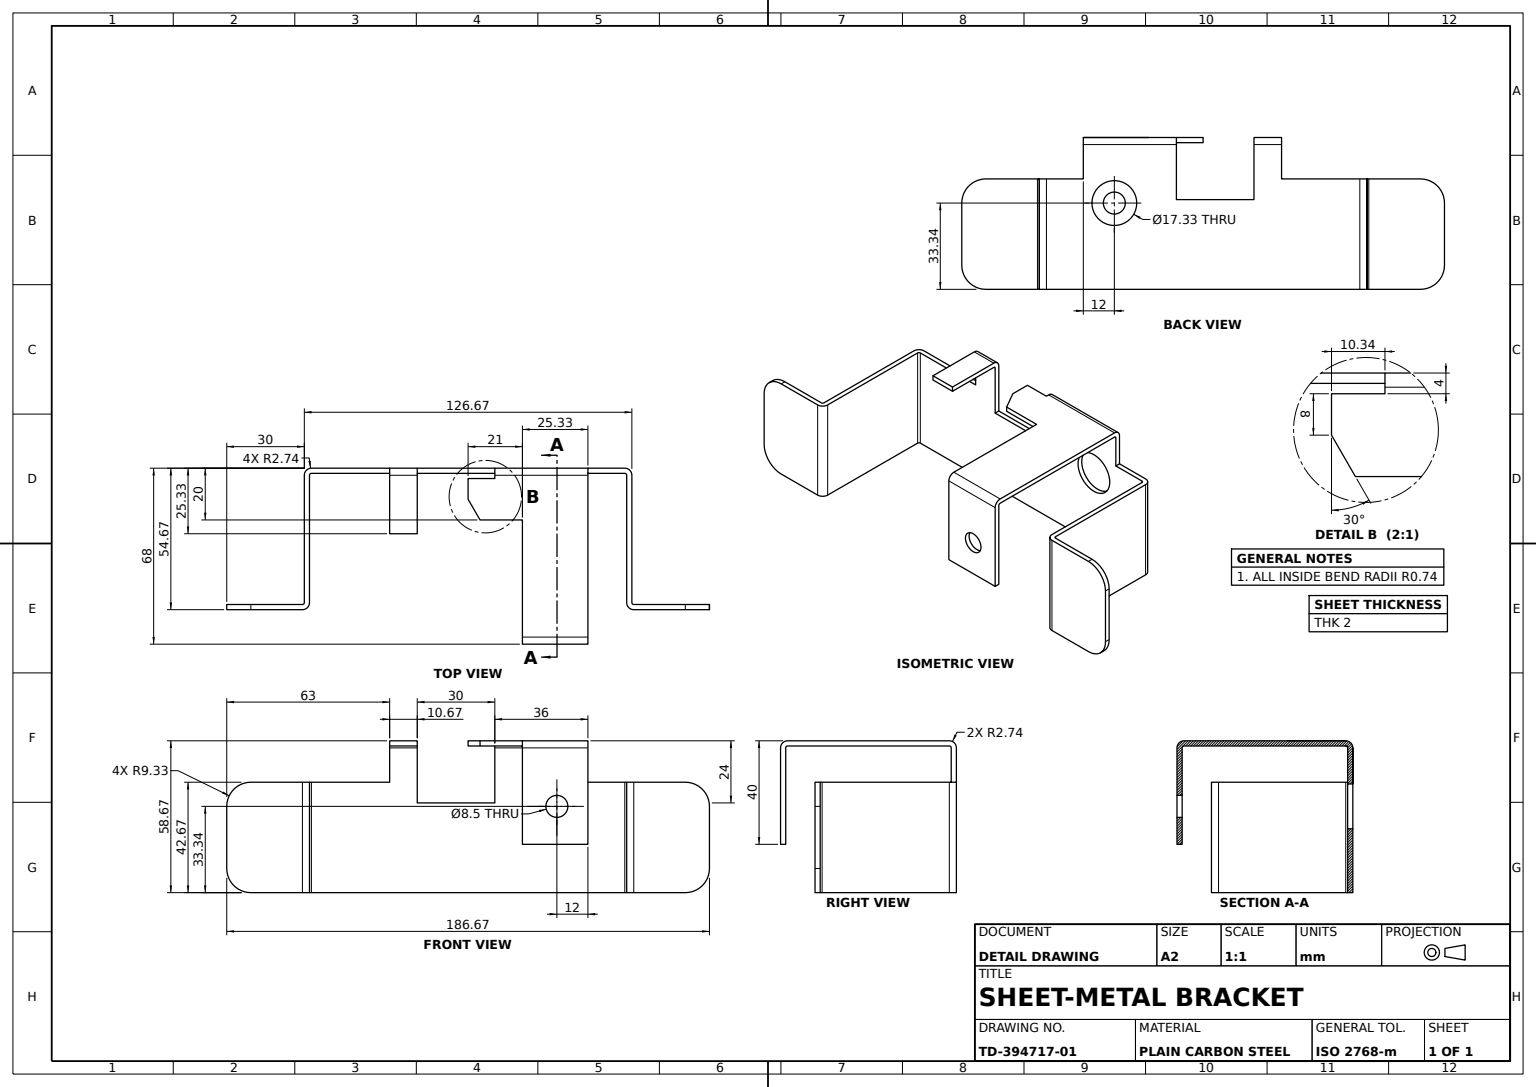
solid
v1 (10.335,13.335,-2)
v2 (10.335,13.335,0)
e1 v1 v2 LINE
v3 (-19.665,13.335,-2)
e2 v1 v3 LINE
v4 (-19.665,13.335,0)
e3 v3 v4 LINE
e4 v4 v2 LINE
face PLANE(AX(P(10.335,13.335,-58),D(0,-1,0),D(1,0,0))) rev [-e1 e2 e3 e4]
v5 (63.335,21.335,49.9334)
v6 (64.0716,21.335,50.67)
e5 v5 v6 CIRCLE(AX(P(64.0716,21.335,49.9334),D(0,1,0),D(0,0,-1)),0.7366)
v7 (64.0716,-21.335,50.67)
e6 v6 v7 LINE
v8 (63.335,-21.335,49.9334)
e7 v7 v8 CIRCLE(AX(P(64.0716,-21.335,49.9334),D(0,-1,0),D(0,0,-1)),0.7366)
e8 v8 v5 LINE
face CYL(AX(P(64.0716,-21.335,49.9334),D(0,-1,0),D(0,0,1)),0.7366) rev [e5 e6 e7 e8]
v9 (-84.005,-21.335,52.67)
v10 (-84.005,-21.335,50.67)
e9 v9 v10 LINE
v11 (-93.335,-12.005,52.67)
e10 v11 v9 CIRCLE(AX(P(-84.005,-12.005,52.67),D(0,0,1),D(1,0,0)),9.33)
v12 (-93.335,-12.005,50.67)
e11 v12 v11 LINE
e12 v10 v12 CIRCLE(AX(P(-84.005,-12.005,50.67),D(0,0,-1),D(1,0,0)),9.33)
face CYL(AX(P(-84.005,-12.005,52.67),D(0,0,-1),D(-1,0,0)),9.33) [-e9 -e10 -e11 -e12]
v13 (46.335,34.5984,66)
v14 (21.005,34.5984,66)
e13 v13 v14 LINE
v15 (46.335,37.335,63.2634)
e14 v15 v13 CIRCLE(AX(P(46.335,34.5984,63.2634),D(1,0,0),D(0,0,1)),2.7366)
v16 (21.005,37.335,63.2634)
e15 v16 v15 LINE
e16 v14 v16 CIRCLE(AX(P(21.005,34.5984,63.2634),D(-1,0,0),D(0,0,-1)),2.7366)
face CYL(AX(P(10.335,34.5984,63.2634),D(-1,0,0),D(0,0,1)),2.7366) [-e13 -e14 -e15 -e16]
v17 (38.585,12.005,64)
v18 (38.585,12.005,66)
e17 v17 v18 LINE
v19 (30.085,12.005,66)
e18 v18 v19 CIRCLE(AX(P(34.335,12.005,66),D(0,0,1),D(1,0,0)),4.25)
v20 (30.085,12.005,64)
e19 v20 v19 LINE
e20 v17 v20 CIRCLE(AX(P(34.335,12.005,64),D(0,0,1),D(0,-1,0)),4.25)
face CYL(AX(P(34.335,12.005,62),D(0,0,1),D(1,0,0)),4.25) rev [e17 e18 -e19 -e20]
v21 (61.335,21.335,0.7366)
v22 (60.5984,21.335,0)
e21 v21 v22 CIRCLE(AX(P(60.5984,21.335,0.7366),D(0,1,0),D(0,0,1)),0.7366)
v23 (63.335,21.335,0.7366)
e22 v21 v23 LINE
v24 (60.5984,21.335,-2)
e23 v23 v24 CIRCLE(AX(P(60.5984,21.335,0.7366),D(0,1,0),D(0,0,1)),2.7366)
e24 v22 v24 LINE
face PLANE(AX(P(60.5984,21.335,0.7366),D(0,-1,0),D(0,0,-1))) rev [-e21 e22 e23 -e24]
v25 (-64.0716,-21.335,50.67)
e25 v25 v10 LINE
v26 (-93.335,12.005,50.67)
e26 v12 v26 LINE
v27 (-84.005,21.335,50.67)
e27 v26 v27 CIRCLE(AX(P(-84.005,12.005,50.67),D(0,0,-1),D(1,0,0)),9.33)
v28 (-64.0716,21.335,50.67)
e28 v27 v28 LINE
e29 v25 v28 LINE
face PLANE(AX(P(0,0,50.67),D(0,0,1),D(1,0,0))) rev [e25 e12 e26 e27 e28 -e29]
v29 (-30.335,37.335,0.7366)
v30 (-30.335,37.335,23.33)
e30 v29 v30 LINE
v31 (-19.665,37.335,23.33)
e31 v30 v31 LINE
v32 (-19.665,37.335,0.7366)
e32 v31 v32 LINE
e33 v29 v32 LINE
face PLANE(AX(P(0,37.335,0),D(0,-1,0),D(0,0,-1))) rev [e30 e31 e32 -e33]
v33 (-84.005,21.335,52.67)
e34 v27 v33 LINE
v34 (-93.335,12.005,52.67)
e35 v34 v26 LINE
e36 v33 v34 CIRCLE(AX(P(-84.005,12.005,52.67),D(0,0,1),D(1,0,0)),9.33)
face CYL(AX(P(-84.005,12.005,52.67),D(0,0,-1),D(-1,0,0)),9.33) [-e34 -e27 -e35 -e36]
v35 (61.335,21.335,49.9334)
e37 v21 v35 LINE
e38 v5 v35 LINE
e39 v23 v5 LINE
face PLANE(AX(P(63.335,21.335,52.67),D(0,-1,0),D(0,0,-1))) rev [e37 -e38 -e39 -e22]
v36 (25.67,12.005,-2)
v37 (43,12.005,-2)
e40 v36 v37 CIRCLE(AX(P(34.335,12.005,-2),D(0,0,-1),D(-1,0,0)),8.665)
e41 v37 v36 CIRCLE(AX(P(34.335,12.005,-2),D(0,0,-1),D(-1,0,0)),8.665)
v38 (10.335,34.5984,-2)
v39 (46.335,34.5984,-2)
e42 v38 v39 LINE
v40 (46.335,21.335,-2)
e43 v40 v39 LINE
e44 v24 v40 LINE
v41 (60.5984,-21.335,-2)
e45 v24 v41 LINE
v42 (-60.5984,-21.335,-2)
e46 v42 v41 LINE
v43 (-60.5984,21.335,-2)
e47 v42 v43 LINE
v44 (-30.335,21.335,-2)
e48 v44 v43 LINE
v45 (-30.335,34.5984,-2)
e49 v45 v44 LINE
v46 (-19.665,34.5984,-2)
e50 v45 v46 LINE
e51 v3 v46 LINE
e52 v38 v1 LINE
face PLANE(AX(P(0,0,-2),D(0,0,-1),D(-1,0,0))) [-e40 -e41] [e42 -e43 -e44 e45 -e46 e47 -e48 -e49 e50 -e51 -e2 -e52]
v47 (10.335,37.335,0.7366)
v48 (46.335,37.335,0.7366)
e53 v47 v48 LINE
v49 (10.335,37.335,2)
e54 v49 v47 LINE
v50 (0,37.335,2)
e55 v50 v49 LINE
v51 (0,37.335,10)
e56 v51 v50 LINE
v52 (4.618802,37.335,18)
e57 v51 v52 LINE
v53 (21.005,37.335,18)
e58 v53 v52 LINE
e59 v53 v16 LINE
e60 v15 v48 LINE
face PLANE(AX(P(0,37.335,0),D(0,-1,0),D(0,0,-1))) rev [-e53 -e54 -e55 -e56 e57 -e58 e59 e15 e60]
v54 (93.335,12.005,52.67)
v55 (84.005,21.335,52.67)
e61 v54 v55 CIRCLE(AX(P(84.005,12.005,52.67),D(0,0,1),D(-1,0,0)),9.33)
v56 (64.0716,21.335,52.67)
e62 v55 v56 LINE
v57 (64.0716,-21.335,52.67)
e63 v57 v56 LINE
v58 (84.005,-21.335,52.67)
e64 v57 v58 LINE
v59 (93.335,-12.005,52.67)
e65 v58 v59 CIRCLE(AX(P(84.005,-12.005,52.67),D(0,0,1),D(-1,0,0)),9.33)
e66 v59 v54 LINE
face PLANE(AX(P(0,0,52.67),D(0,0,-1),D(-1,0,0))) rev [e61 e62 -e63 e64 e65 e66]
v60 (0,35.335,2)
e67 v50 v60 LINE
v61 (0,35.335,10)
e68 v61 v60 LINE
e69 v61 v51 LINE
face PLANE(AX(P(0,37.335,8),D(-1,0,0),D(0,0,1))) [e67 -e68 e69 e56]
v62 (46.335,21.335,0)
e70 v40 v62 LINE
e71 v22 v62 LINE
face PLANE(AX(P(-63.335,21.335,-2),D(0,1,0),D(0,0,1))) [e24 e44 e70 -e71]
v63 (-61.335,-21.335,0.7366)
v64 (-61.335,-21.335,49.9334)
e72 v63 v64 LINE
v65 (-63.335,-21.335,49.9334)
e73 v65 v64 LINE
v66 (-63.335,-21.335,0.7366)
e74 v66 v65 LINE
e75 v63 v66 LINE
face PLANE(AX(P(-63.335,-21.335,52.67),D(0,1,0),D(0,0,1))) rev [e72 -e73 -e74 -e75]
v67 (93.335,-12.005,50.67)
e76 v59 v67 LINE
v68 (93.335,12.005,50.67)
e77 v67 v68 LINE
e78 v68 v54 LINE
face PLANE(AX(P(93.335,21.335,52.67),D(-1,0,0),D(0,0,1))) rev [e76 e77 e78 -e66]
v69 (-63.335,21.335,49.9334)
e79 v69 v65 LINE
v70 (-63.335,21.335,0.7366)
e80 v69 v70 LINE
e81 v66 v70 LINE
face PLANE(AX(P(-63.335,0,0),D(1,0,0),D(0,0,-1))) rev [e74 -e79 e80 -e81]
v71 (43,12.005,0)
e82 v37 v71 LINE
v72 (25.67,12.005,0)
e83 v71 v72 CIRCLE(AX(P(34.335,12.005,0),D(0,0,1),D(1,0,0)),8.665)
e84 v36 v72 LINE
face CYL(AX(P(34.335,12.005,-10.67),D(0,0,1),D(1,0,0)),8.665) rev [e40 e82 e83 -e84]
e85 v29 v45 CIRCLE(AX(P(-30.335,34.5984,0.7366),D(-1,0,0),D(0,0,1)),2.7366)
e86 v46 v32 CIRCLE(AX(P(-19.665,34.5984,0.7366),D(1,0,0),D(0,0,1)),2.7366)
face CYL(AX(P(-30.335,34.5984,0.7366),D(-1,0,0),D(0,1,0)),2.7366) [-e50 -e85 e33 -e86]
v73 (-64.0716,-21.335,52.67)
e87 v64 v73 CIRCLE(AX(P(-64.0716,-21.335,49.9334),D(0,-1,0),D(0,0,1)),2.7366)
e88 v25 v73 LINE
e89 v65 v25 CIRCLE(AX(P(-64.0716,-21.335,49.9334),D(0,-1,0),D(0,0,1)),0.7366)
face PLANE(AX(P(-64.0716,-21.335,49.9334),D(0,-1,0),D(0,0,-1))) [e73 e87 -e88 -e89]
v74 (46.335,35.335,0.7366)
v75 (10.335,35.335,0.7366)
e90 v74 v75 LINE
v76 (46.335,35.335,63.2634)
e91 v76 v74 LINE
v77 (21.005,35.335,63.2634)
e92 v77 v76 LINE
v78 (21.005,35.335,18)
e93 v78 v77 LINE
v79 (4.618802,35.335,18)
e94 v79 v78 LINE
e95 v79 v61 LINE
v80 (10.335,35.335,2)
e96 v60 v80 LINE
e97 v75 v80 LINE
face PLANE(AX(P(0,35.335,0),D(0,-1,0),D(0,0,-1))) [-e90 -e91 -e92 -e93 -e94 e95 e68 e96 -e97]
v81 (63.335,-21.335,0.7366)
e98 v23 v81 LINE
e99 v41 v81 CIRCLE(AX(P(60.5984,-21.335,0.7366),D(0,-1,0),D(0,0,1)),2.7366)
face CYL(AX(P(60.5984,21.335,0.7366),D(0,1,0),D(1,0,0)),2.7366) [-e23 e98 -e99 -e45]
e100 v20 v17 CIRCLE(AX(P(34.335,12.005,64),D(0,0,1),D(0,-1,0)),4.25)
e101 v19 v18 CIRCLE(AX(P(34.335,12.005,66),D(0,0,1),D(1,0,0)),4.25)
face CYL(AX(P(34.335,12.005,62),D(0,0,1),D(1,0,0)),4.25) rev [-e17 -e100 e19 e101]
e102 v52 v79 LINE
face PLANE(AX(P(4.618802,0,18),D(0.866025404,0,-0.5),D(0,-1,0))) rev [-e95 -e102 -e57 -e69]
e103 v28 v69 CIRCLE(AX(P(-64.0716,21.335,49.9334),D(0,1,0),D(0,0,1)),0.7366)
face CYL(AX(P(-64.0716,21.335,49.9334),D(0,1,0),D(0,0,1)),0.7366) rev [e29 e103 e79 e89]
v82 (84.005,-21.335,50.67)
e104 v7 v82 LINE
e105 v82 v58 LINE
e106 v7 v57 LINE
face PLANE(AX(P(93.335,-21.335,52.67),D(0,1,0),D(0,0,1))) rev [e104 e105 -e64 -e106]
v83 (84.005,21.335,50.67)
e107 v55 v83 LINE
e108 v83 v6 LINE
e109 v6 v56 LINE
face PLANE(AX(P(63.335,21.335,52.67),D(0,-1,0),D(0,0,-1))) rev [e107 e108 e109 -e62]
e110 v8 v81 LINE
v84 (61.335,-21.335,49.9334)
e111 v8 v84 LINE
v85 (61.335,-21.335,0.7366)
e112 v84 v85 LINE
e113 v85 v81 LINE
face PLANE(AX(P(63.335,-21.335,0),D(0,1,0),D(0,0,1))) rev [-e110 e111 e112 e113]
e114 v78 v53 LINE
e115 v77 v16 LINE
face PLANE(AX(P(21.005,-2.665,8),D(1,0,0),D(0,0,-1))) rev [-e114 e93 e115 -e59]
v86 (60.5984,-21.335,0)
e116 v86 v85 CIRCLE(AX(P(60.5984,-21.335,0.7366),D(0,-1,0),D(0,0,1)),0.7366)
e117 v86 v41 LINE
face PLANE(AX(P(60.5984,-21.335,0.7366),D(0,-1,0),D(0,0,-1))) [-e113 -e116 e117 e99]
v87 (-60.5984,-21.335,0)
e118 v63 v87 CIRCLE(AX(P(-60.5984,-21.335,0.7366),D(0,-1,0),D(0,0,-1)),0.7366)
v88 (-60.5984,21.335,0)
e119 v87 v88 LINE
v89 (-61.335,21.335,0.7366)
e120 v88 v89 CIRCLE(AX(P(-60.5984,21.335,0.7366),D(0,1,0),D(0,0,-1)),0.7366)
e121 v89 v63 LINE
face CYL(AX(P(-60.5984,-21.335,0.7366),D(0,-1,0),D(-1,0,0)),0.7366) rev [e118 e119 e120 e121]
v90 (-30.335,35.335,23.33)
v91 (-19.665,35.335,23.33)
e122 v90 v91 LINE
v92 (-30.335,35.335,0.7366)
e123 v92 v90 LINE
v93 (-19.665,35.335,0.7366)
e124 v93 v92 LINE
e125 v91 v93 LINE
face PLANE(AX(P(0,35.335,0),D(0,-1,0),D(0,0,-1))) [-e122 -e123 -e124 -e125]
e126 v35 v56 CIRCLE(AX(P(64.0716,21.335,49.9334),D(0,1,0),D(0,0,-1)),2.7366)
face PLANE(AX(P(64.0716,21.335,49.9334),D(0,1,0),D(0,0,1))) [e126 -e109 -e5 e38]
e127 v31 v91 LINE
e128 v30 v90 LINE
face PLANE(AX(P(-19.665,37.335,23.33),D(0,0,-1),D(0,1,0))) rev [-e127 -e31 e128 e122]
e129 v43 v70 CIRCLE(AX(P(-60.5984,21.335,0.7366),D(0,1,0),D(0,0,-1)),2.7366)
e130 v66 v42 CIRCLE(AX(P(-60.5984,-21.335,0.7366),D(0,-1,0),D(0,0,-1)),2.7366)
face CYL(AX(P(-60.5984,-21.335,0.7366),D(0,-1,0),D(-1,0,0)),2.7366) [e81 -e129 -e47 -e130]
v94 (-30.335,21.335,0)
e131 v44 v94 LINE
v95 (-30.335,34.5984,0)
e132 v95 v94 LINE
e133 v95 v45 LINE
face PLANE(AX(P(-30.335,21.335,-2),D(-1,0,0),D(0,0,1))) [e49 e131 -e132 e133]
v96 (46.335,-2.665,66)
v97 (46.335,-2.665,64)
e134 v96 v97 LINE
v98 (21.005,-2.665,66)
e135 v96 v98 LINE
v99 (21.005,-2.665,64)
e136 v99 v98 LINE
e137 v97 v99 LINE
face PLANE(AX(P(10.335,-2.665,66),D(0,-1,0),D(0,0,-1))) [-e134 e135 -e136 -e137]
e138 v83 v68 CIRCLE(AX(P(84.005,12.005,50.67),D(0,0,-1),D(-1,0,0)),9.33)
face CYL(AX(P(84.005,12.005,52.67),D(0,0,-1),D(-1,0,0)),9.33) [-e107 -e61 -e78 -e138]
v100 (46.335,34.5984,64)
e139 v100 v13 LINE
e140 v76 v100 CIRCLE(AX(P(46.335,34.5984,63.2634),D(1,0,0),D(0,0,1)),0.7366)
e141 v76 v15 LINE
face PLANE(AX(P(46.335,34.5984,63.2634),D(1,0,0),D(0,0,-1))) [-e139 -e140 e141 e14]
v101 (-64.0716,21.335,52.67)
e142 v73 v101 LINE
e143 v33 v101 LINE
e144 v11 v34 LINE
e145 v73 v9 LINE
face PLANE(AX(P(0,0,52.67),D(0,0,1),D(1,0,0))) [e142 -e143 e36 -e144 e10 -e145]
v102 (21.005,34.5984,64)
e146 v102 v77 CIRCLE(AX(P(21.005,34.5984,63.2634),D(-1,0,0),D(0,0,-1)),0.7366)
e147 v14 v102 LINE
face PLANE(AX(P(21.005,-2.665,8),D(1,0,0),D(0,0,-1))) rev [e16 -e115 -e146 -e147]
e148 v84 v35 LINE
e149 v57 v84 CIRCLE(AX(P(64.0716,-21.335,49.9334),D(0,-1,0),D(0,0,-1)),2.7366)
face CYL(AX(P(64.0716,-21.335,49.9334),D(0,-1,0),D(0,0,1)),2.7366) [-e148 -e149 e63 -e126]
face PLANE(AX(P(0,0,18),D(0,0,1),D(1,0,0))) [e114 e58 e102 e94]
e150 v92 v29 LINE
face PLANE(AX(P(-30.335,37.335,23.33),D(1,0,0),D(0,0,-1))) rev [-e150 e123 -e128 -e30]
v103 (-19.665,34.5984,0)
e151 v103 v93 CIRCLE(AX(P(-19.665,34.5984,0.7366),D(1,0,0),D(0,0,1)),0.7366)
e152 v92 v95 CIRCLE(AX(P(-30.335,34.5984,0.7366),D(-1,0,0),D(0,0,1)),0.7366)
e153 v95 v103 LINE
face CYL(AX(P(-30.335,34.5984,0.7366),D(-1,0,0),D(0,1,0)),0.7366) rev [e151 e124 e152 e153]
e154 v67 v82 CIRCLE(AX(P(84.005,-12.005,50.67),D(0,0,-1),D(-1,0,0)),9.33)
face CYL(AX(P(84.005,-12.005,52.67),D(0,0,-1),D(-1,0,0)),9.33) [-e65 -e105 -e154 -e76]
v104 (-61.335,21.335,49.9334)
e155 v69 v104 LINE
e156 v104 v89 LINE
e157 v89 v70 LINE
face PLANE(AX(P(-63.335,21.335,0),D(0,-1,0),D(0,0,-1))) rev [e155 e156 e157 -e80]
e158 v100 v97 LINE
e159 v13 v96 LINE
face PLANE(AX(P(46.335,-2.665,66),D(1,0,0),D(0,0,-1))) [-e158 e139 e159 e134]
e160 v28 v101 LINE
e161 v101 v104 CIRCLE(AX(P(-64.0716,21.335,49.9334),D(0,1,0),D(0,0,1)),2.7366)
face PLANE(AX(P(-64.0716,21.335,49.9334),D(0,-1,0),D(0,0,-1))) rev [e160 e161 -e155 -e103]
e162 v87 v86 LINE
e163 v87 v42 LINE
face PLANE(AX(P(-63.335,-21.335,-2),D(0,-1,0),D(0,0,-1))) [e46 -e117 -e162 e163]
e164 v85 v21 LINE
e165 v22 v86 LINE
face CYL(AX(P(60.5984,21.335,0.7366),D(0,1,0),D(1,0,0)),0.7366) rev [e116 e164 e21 e165]
v105 (46.335,34.5984,0)
e166 v62 v105 LINE
e167 v105 v39 LINE
face PLANE(AX(P(46.335,21.335,-2),D(1,0,0),D(0,0,-1))) [-e166 -e70 e43 -e167]
e168 v72 v71 CIRCLE(AX(P(34.335,12.005,0),D(0,0,1),D(1,0,0)),8.665)
face CYL(AX(P(34.335,12.005,-10.67),D(0,0,1),D(1,0,0)),8.665) rev [e168 -e82 e41 e84]
e169 v103 v46 LINE
e170 v103 v4 LINE
face PLANE(AX(P(-19.665,37.335,-58),D(-1,0,0),D(0,-1,0))) rev [-e169 e170 -e3 e51]
e171 v93 v32 LINE
face PLANE(AX(P(-19.665,37.335,0),D(-1,0,0),D(0,0,1))) rev [-e32 e127 e125 e171]
face PLANE(AX(P(-93.335,21.335,52.67),D(-1,0,0),D(0,0,1))) [e11 e144 e35 -e26]
face PLANE(AX(P(61.335,0,0),D(-1,0,0),D(0,0,1))) [-e112 e148 -e37 -e164]
e172 v94 v88 LINE
e173 v88 v43 LINE
face PLANE(AX(P(-63.335,21.335,-2),D(0,1,0),D(0,0,1))) [-e172 -e131 e48 -e173]
v106 (10.335,34.5984,0)
e174 v106 v105 LINE
e175 v106 v2 LINE
face PLANE(AX(P(0,0,0),D(0,0,-1),D(-1,0,0))) rev [-e168 -e83] [e132 e172 -e119 e162 -e165 e71 e166 -e174 e175 -e4 -e170 -e153]
e176 v47 v38 CIRCLE(AX(P(10.335,34.5984,0.7366),D(-1,0,0),D(0,0,1)),2.7366)
e177 v106 v75 CIRCLE(AX(P(10.335,34.5984,0.7366),D(1,0,0),D(0,0,1)),0.7366)
e178 v80 v49 LINE
face PLANE(AX(P(10.335,21.335,-2),D(-1,0,0),D(0,0,1))) [e176 e52 e1 -e175 e177 e97 e178 e54]
e179 v100 v102 LINE
face CYL(AX(P(10.335,34.5984,63.2634),D(-1,0,0),D(0,0,1)),0.7366) rev [e179 e146 e92 e140]
face PLANE(AX(P(-60.5984,21.335,0.7366),D(0,1,0),D(0,0,1))) [-e157 -e120 e173 e129]
e180 v39 v48 CIRCLE(AX(P(46.335,34.5984,0.7366),D(1,0,0),D(0,0,1)),2.7366)
face CYL(AX(P(10.335,34.5984,0.7366),D(-1,0,0),D(0,1,0)),2.7366) [-e176 e53 -e180 -e42]
face PLANE(AX(P(-60.5984,-21.335,0.7366),D(0,1,0),D(0,0,1))) rev [e75 e130 -e163 -e118]
e181 v104 v64 LINE
face PLANE(AX(P(-61.335,0,0),D(1,0,0),D(0,0,-1))) [-e121 -e156 e181 -e72]
face PLANE(AX(P(63.335,0,0),D(-1,0,0),D(0,0,1))) rev [e39 -e8 e110 -e98]
face PLANE(AX(P(64.0716,-21.335,49.9334),D(0,1,0),D(0,0,1))) rev [-e111 -e7 e106 e149]
face PLANE(AX(P(-19.665,34.5984,0.7366),D(1,0,0),D(0,0,-1))) [e86 -e171 -e151 e169]
face PLANE(AX(P(-30.335,34.5984,0.7366),D(1,0,0),D(0,0,-1))) rev [e150 e85 -e133 -e152]
face PLANE(AX(P(0,0,50.67),D(0,0,-1),D(-1,0,0))) [-e77 e154 -e104 -e6 -e108 e138]
face PLANE(AX(P(-93.335,-21.335,52.67),D(0,-1,0),D(0,0,-1))) [e145 e9 -e25 e88]
e182 v99 v102 LINE
e183 v98 v14 LINE
face PLANE(AX(P(21.005,-2.665,8),D(1,0,0),D(0,0,-1))) rev [-e182 e136 e183 e147]
face PLANE(AX(P(0,0,66),D(0,0,1),D(0,-1,0))) [-e135 -e159 e13 -e183] [-e18 -e101]
face PLANE(AX(P(-63.335,21.335,52.67),D(0,1,0),D(0,0,1))) [e34 e143 -e160 -e28]
e184 v105 v74 CIRCLE(AX(P(46.335,34.5984,0.7366),D(1,0,0),D(0,0,1)),0.7366)
face CYL(AX(P(10.335,34.5984,0.7366),D(-1,0,0),D(0,1,0)),0.7366) rev [-e177 e174 e184 e90]
face PLANE(AX(P(0,35.335,2),D(0,0,1),D(1,0,0))) rev [-e178 -e96 -e67 e55]
face PLANE(AX(P(0,0,64),D(0,0,1),D(0,-1,0))) rev [e158 e137 e182 -e179] [e100 e20]
e185 v74 v48 LINE
face PLANE(AX(P(46.335,37.335,0),D(-1,0,0),D(0,0,1))) rev [e185 -e60 -e141 e91]
face PLANE(AX(P(46.335,34.5984,0.7366),D(1,0,0),D(0,0,-1))) [e180 -e185 -e184 e167]
face CYL(AX(P(-64.0716,21.335,49.9334),D(0,1,0),D(0,0,1)),2.7366) [-e142 -e87 -e181 -e161]
